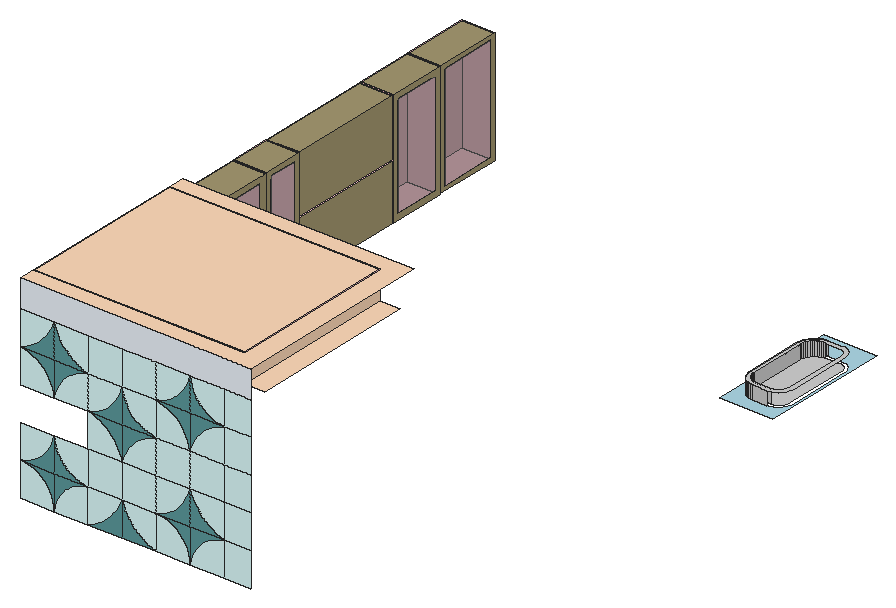
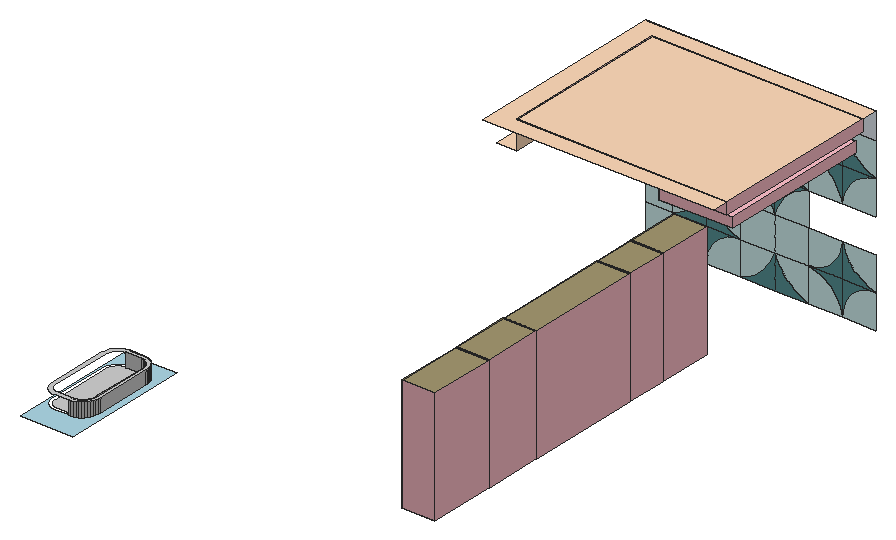
# SketchUp Ruby script. Lengths in inches.
U = 1.inch
M = Sketchup.active_model
def pt(a) = Geom::Point3d.new(a.map { |v| v * U })
def face(e, loops, mat)
  f = e.add_face(loops[0].map { |a| pt(a) })
  loops[1..].each { |l| e.add_face(l.map { |a| pt(a) }).erase! }
  f.material = f.back_material = mat if mat
  f
end
# faces: each face lists its corners as indices into pts; further lists are holes
def faces(e, pts, list, mat = nil) = list.each { |f| face(e, (f[0].is_a?(Array) ? f : [f]).map { |l| l.map { |i| pts[i] } }, mat) }
# xy, xz, yz: faces in a plane at the given z, y or x. An outline is a flat list of corners, or four numbers for a rectangle; further outlines are holes
def ring(l) = l.size == 4 ? [[l[0], l[1]], [l[2], l[1]], [l[2], l[3]], [l[0], l[3]]] : l.each_slice(2).to_a
def flat(e, list, mat, &to3) = list.each { |f| face(e, (f[0].is_a?(Array) ? f : [f]).map { |l| ring(l).map { |u, v| to3.(u, v) } }, mat) }
def xy(e, z, list, mat = nil) = flat(e, list, mat) { |x, y| [x, y, z] }
def xz(e, y, list, mat = nil) = flat(e, list, mat) { |x, z| [x, y, z] }
def yz(e, x, list, mat = nil) = flat(e, list, mat) { |y, z| [x, y, z] }
def lines(e, pts, list) = list.each { |a, b| e.add_line(pt(pts[a]), pt(pts[b])) }
# prism: a flat outline (further loops are holes) pulled along v
def prism(e, loops, v, mat = nil)
  f = face(e, loops, mat); d = Geom::Vector3d.new(v.map { |x| x * U })
  f.pushpull(f.normal.samedirection?(d) ? d.length : -d.length)
end
def box(e, o, s, mat = nil) = prism(e, [[o, [o[0] + s[0], o[1], o[2]], [o[0] + s[0], o[1] + s[1], o[2]], [o[0], o[1] + s[1], o[2]]]], [0, 0, s[2]], mat)
def at(x, y, z, deg = 0) = Geom::Transformation.translation(pt([x, y, z])) * Geom::Transformation.rotation(ORIGIN, Z_AXIS, deg.degrees)
def axes(o, x, y, z) = Geom::Transformation.new([*x, 0, *y, 0, *z, 0, *pt(o).to_a, 1])
def part(name) = M.definitions.add(name)
# library, detail: a bought-in or finely detailed component or shape, given as its bounding box
def library(name, o, s) = part(name).tap { |d| box(d.entities, o, s) }
def detail(e, o, s) = box(e.add_group.entities, o, s)
def put(e, d, t, mat = nil) = e.add_instance(d, t).tap { |i| i.material = mat if mat }
def group(e, t, mat = nil) = e.add_group.tap { |g| g.transformation = t; g.material = mat if mat }.entities
root = M.entities
M.materials.add("[0006_Pink]").color = [255, 192, 203]
M.materials.add("[0027_PeachPuff]").color = [255, 218, 185]
M.materials.add("[0081_CadetBlue]").color = [95, 158, 160]
M.materials.add("[0090_LightCyan]").color = [224, 255, 255]
M.materials.add("[0093_AliceBlue]").color = [240, 248, 255]
M.materials.add("[0095_LightBlue]").color = [173, 216, 230]
M.materials.add("[Carrera Marble]").color = [207, 207, 207]
M.materials.add("[Translucent Glass Gray]").color = [128, 128, 128]
M.materials["[Translucent Glass Gray]"].alpha = 0.5
M.materials.add("[Wood Lumber ButtJoined]").color = [164, 152, 112]
box(root,[118.5625,343,111.75],[25.9375,54.56,3.75],"[0006_Pink]")
xy(root,60.5,[[[244.5625,486.17,263.2,531.9375],[252.11,491,251.42,491.05,250.75,491.2,250.09,491.4375,249.47,491.77,248.9,492.19,248.38,492.68,247.92,493.24,247.54,493.87,247.24,494.54,247.01,495.25,246.88,495.99,246.83,496.73,246.83,516.85,246.88,517.71,247.04,518.55,247.29,519.36,247.64,520.13,248.08,520.85,248.6,521.49,249.2,522.06,249.86,522.53,250.5625,522.91,251.3125,523.19,252.09,523.36,252.88,523.41,258.18,523.41,258.75,523.37,259.3125,523.25,259.86,523.05,260.37,522.78,260.85,522.43,261.28,522.02,261.66,521.55,261.98,521.03,262.23,520.47,262.41,519.88,262.53,519.27,262.5625,518.65,262.5625,496.67,262.52,495.93,262.39,495.21,262.17,494.5,261.86,493.84,261.48,493.22,261.03,492.66,260.52,492.17,259.95,491.76,259.34,491.43,258.69,491.19,258.02,491.05,257.34,491]]],"[0095_LightBlue]")
xy(root,60.5,[[252.11,492.42,257.34,492.42,257.85,492.45,258.35,492.5625,258.84,492.74,259.3,492.99,259.73,493.3,260.11,493.66,260.45,494.08,260.73,494.54,260.96,495.04,261.125,495.57,261.23,496.12,261.26,496.67,261.26,518.65,261.23,519.09,261.15,519.52,261.03,519.93,260.85,520.32,260.62,520.6875,260.36,521.02,260.05,521.31,259.72,521.55,259.36,521.74,258.97,521.88,258.58,521.97,258.18,522,252.88,522,252.26,521.95,251.65,521.82,251.0625,521.61,250.51,521.31,249.99,520.93,249.53,520.49,249.12,519.98,248.77,519.42,248.5,518.82,248.3,518.18,248.18,517.52,248.14,516.85,248.14,496.73,248.17,496.17,248.27,495.62,248.44,495.08,248.67,494.57,248.96,494.11,249.3,493.68,249.69,493.31,250.125,492.99,250.59,492.74,251.08,492.5625,251.59,492.45]],"[Carrera Marble]")
xy(root,65.34,[[[252.11,491,257.34,491,258.02,491.05,258.69,491.19,259.34,491.43,259.95,491.76,260.52,492.17,261.03,492.66,261.48,493.22,261.86,493.84,262.17,494.5,262.39,495.21,262.52,495.93,262.5625,496.67,262.5625,518.65,262.53,519.27,262.41,519.88,262.23,520.47,261.98,521.03,261.66,521.55,261.28,522.02,260.85,522.43,260.37,522.78,259.86,523.05,259.3125,523.25,258.75,523.37,258.18,523.41,252.88,523.41,252.09,523.36,251.3125,523.19,250.5625,522.91,249.86,522.53,249.2,522.06,248.6,521.49,248.08,520.85,247.64,520.13,247.29,519.36,247.04,518.55,246.88,517.71,246.83,516.85,246.83,496.73,246.88,495.99,247.01,495.25,247.24,494.54,247.54,493.87,247.92,493.24,248.38,492.68,248.9,492.19,249.47,491.77,250.09,491.4375,250.75,491.2,251.42,491.05],[252.11,492.42,251.59,492.45,251.08,492.5625,250.59,492.74,250.125,492.99,249.69,493.31,249.3,493.68,248.96,494.11,248.67,494.57,248.44,495.08,248.27,495.62,248.17,496.17,248.14,496.73,248.14,516.85,248.18,517.52,248.3,518.18,248.5,518.82,248.77,519.42,249.12,519.98,249.53,520.49,249.99,520.93,250.51,521.31,251.0625,521.61,251.65,521.82,252.26,521.95,252.88,522,258.18,522,258.58,521.97,258.97,521.88,259.36,521.74,259.72,521.55,260.05,521.31,260.36,521.02,260.62,520.6875,260.85,520.32,261.03,519.93,261.15,519.52,261.23,519.09,261.26,518.65,261.26,496.67,261.23,496.12,261.125,495.57,260.96,495.04,260.73,494.54,260.45,494.08,260.11,493.66,259.73,493.3,259.3,492.99,258.84,492.74,258.35,492.5625,257.85,492.45,257.34,492.42]]],"[Carrera Marble]")
xy(root,76.6875,[[130.1875,408.86,118.5625,408.875,118.58,427.81,130.21,427.8],[130.21,428.36,118.5625,428.375,118.58,442.66,130.23,442.64],[130.22,443.12,118.56,443.125,118.58,483.93,130.24,483.92],[130.25,484.43,118.5625,484.4375,118.58,505.08,130.27,505.06]],"[0006_Pink]")
xy(root,76.84,[[118.5625,505.5625,130.26,529.25]],"[0006_Pink]")
xy(root,96.47,[[129.35,443.12,130.22,443.12,130.24,483.92,129.37,483.93]],"[0006_Pink]")
xy(root,96.97,[[129.35,443.12,129.37,483.93,130.24,483.92,130.22,443.12]],"[0006_Pink]")
xy(root,111.25,[[193.07,339.9375,200.19,399.9375]],"[0027_PeachPuff]")
xy(root,116.9375,[[118.5625,339.9375,193.07,399.9375]],"[0006_Pink]")
xy(root,117.25,[[130.1875,408.86,130.21,427.8,118.58,427.81,118.5625,408.875],[130.21,428.36,130.23,442.64,118.58,442.66,118.5625,428.375],[130.22,443.12,130.24,483.92,118.58,483.93,118.56,443.125],[130.25,484.43,130.27,505.06,118.58,505.08,118.5625,484.4375],[118.5625,505.5625,130.26,529.25]],"[Wood Lumber ButtJoined]")
xy(root,121.1875,[[118.5625,333.9375,200.19,333.9375,200.19,405.9375,118.5625,405.9375,118.5625,399.9375,193.07,399.9375,193.07,339.9375,118.5625,339.9375],[118.5625,339.9375,193.07,399.9375]],"[0027_PeachPuff]")
xz(root,333.9375,[[130.5625,51.41,130.5625,63.41,118.5625,63.41,120.14,63.34,121.69,63.05,123.2,62.57,124.62,61.88,125.9375,61.01,127.125,59.97,128.16,58.78,129.03,57.46,129.72,56.04,130.21,54.54,130.49,52.99],[130.5625,51.41,130.83,52.91,131.26,54.37,131.84,55.78,132.59,57.11,133.47,58.35,134.49,59.49,135.62,60.5,136.86,61.39,138.19,62.125,139.6,62.71,141.0625,63.14,142.5625,63.41,130.5625,63.41],[142.5625,51.41,154.5625,51.41,154.5625,63.41,154.01,62.06,153.36,60.75,152.62,59.49,151.79,58.3,150.875,57.16,149.88,56.09,148.8125,55.1,147.68,54.18,146.48,53.35,145.22,52.61,143.91,51.96],[154.5625,51.41,166.5625,51.41,165.18,51.91,163.85,52.52,162.5625,53.23,161.34,54.05,160.18,54.95,159.1,55.95,158.11,57.03,157.2,58.18,156.39,59.41,155.67,60.69,155.0625,62.03,154.5625,63.41],[178.5625,51.41,178.5625,63.41,166.5625,63.41,168.15,63.35,169.71,63.09,171.22,62.61,172.65,61.93,173.98,61.06,175.17,60.02,176.21,58.82,177.08,57.5,177.76,56.0625,178.24,54.55,178.51,52.99],
  [178.5625,51.41,178.9,52.88,179.38,54.3,180,55.68,180.76,56.97,181.65,58.19,182.66,59.31,183.78,60.32,185,61.21,186.3,61.97,187.67,62.59,189.09,63.07,190.5625,63.41,178.5625,63.41],[118.5625,63.41,130.5625,63.41,130.5625,75.41,130.2,73.96,129.6875,72.55,129.05,71.19,128.27,69.91,127.38,68.71,126.375,67.6,125.26,66.59,124.0625,65.7,122.78,64.93,121.42,64.28,120.01,63.78],[130.5625,63.41,142.5625,63.41,141.02,63.57,139.51,63.92,138.05,64.45,136.67,65.16,135.38,66.04,134.22,67.07,133.19,68.23,132.32,69.51,131.61,70.89,131.07,72.35,130.72,73.86,130.5625,75.41],[166.5625,63.41,178.5625,63.41,178.5625,75.41,178.16,73.97,177.63,72.58,176.97,71.25,176.1875,69.98,175.29,68.79,174.29,67.68,173.18,66.68,171.99,65.78,170.73,65,169.39,64.34,168,63.81],[178.5625,63.41,190.5625,63.41,189.19,63.93,187.86,64.55,186.59,65.27,185.37,66.09,184.22,67,183.15,67.99,182.15,69.07,181.24,70.22,180.42,71.43,179.7,72.71,179.08,74.04,178.5625,75.41],
  [154.5625,75.41,154.5625,87.41,142.5625,87.41,143.98,86.97,145.35,86.41,146.67,85.74,147.93,84.94,149.1,84.04,150.2,83.04,151.2,81.95,152.1,80.77,152.89,79.52,153.57,78.2,154.13,76.83],[154.5625,75.41,155.01,76.82,155.59,78.18,156.27,79.49,157.07,80.74,157.97,81.91,158.97,83,160.0625,84,161.23,84.9,162.48,85.7,163.79,86.39,165.15,86.96,166.5625,87.41,154.5625,87.41],[130.5625,87.41,130.5625,99.41,118.5625,99.41,120.09,99.2,121.57,98.81,123.01,98.24,124.36,97.52,125.62,96.64,126.77,95.62,127.79,94.47,128.67,93.21,129.4,91.85,129.96,90.42,130.35,88.93],[130.5625,87.41,130.93,88.86,131.4375,90.27,132.08,91.625,132.85,92.91,133.74,94.11,134.75,95.22,135.86,96.23,137.0625,97.12,138.35,97.89,139.7,98.53,141.11,99.04,142.5625,99.41,130.5625,99.41],[142.5625,87.41,154.5625,87.41,154.5625,99.41,154.18,97.96,153.66,96.5625,153.01,95.22,152.23,93.94,151.34,92.75,150.33,91.64,149.22,90.64,148.03,89.74,146.75,88.96,145.41,88.3125,144.01,87.79],
  [154.5625,87.41,166.5625,87.41,165.0625,87.67,163.6,88.1,162.19,88.69,160.86,89.43,159.62,90.31,158.49,91.33,157.47,92.47,156.59,93.71,155.84,95.04,155.26,96.45,154.83,97.91,154.5625,99.41],[178.5625,87.41,178.5625,99.41,166.5625,99.41,168.0625,99.14,169.53,98.71,170.93,98.125,172.26,97.39,173.5,96.5,174.64,95.49,175.66,94.35,176.54,93.11,177.28,91.78,177.87,90.37,178.3,88.91],[178.5625,87.41,179.03,88.81,179.61,90.16,180.31,91.46,181.11,92.7,182.02,93.87,183.02,94.95,184.1,95.95,185.27,96.86,186.51,97.66,187.81,98.36,189.16,98.94,190.5625,99.41,178.5625,99.41],[118.5625,99.41,130.5625,99.41,130.5625,111.41,130.04,110.04,129.42,108.71,128.7,107.43,127.88,106.22,126.97,105.07,125.98,103.99,124.9,103,123.75,102.09,122.54,101.27,121.26,100.55,119.93,99.93],[130.5625,99.41,142.5625,99.41,141.14,99.84,139.77,100.4,138.45,101.08,137.2,101.87,136.02,102.77,134.93,103.77,133.93,104.87,133.03,106.05,132.23,107.3,131.56,108.62,131,109.99,130.5625,111.41],
  [166.5625,99.41,178.5625,99.41,178.5625,111.41,178.2,109.96,177.6875,108.55,177.05,107.19,176.27,105.91,175.38,104.71,174.375,103.6,173.26,102.59,172.0625,101.7,170.78,100.93,169.42,100.28,168.01,99.78],[178.5625,99.41,190.5625,99.41,189.03,99.6,187.54,99.98,186.1,100.53,184.73,101.25,183.46,102.13,182.31,103.15,181.28,104.31,180.41,105.58,179.6875,106.94,179.13,108.38,178.76,109.88,178.5625,111.41]],"[0081_CadetBlue]")
xz(root,333.9375,[[118.5625,51.41,130.5625,51.41,130.49,52.99,130.21,54.54,129.72,56.04,129.03,57.46,128.16,58.78,127.125,59.97,125.9375,61.01,124.62,61.88,123.2,62.57,121.69,63.05,120.14,63.34,118.5625,63.41],[130.5625,51.41,142.5625,51.41,142.5625,63.41,141.0625,63.14,139.6,62.71,138.19,62.125,136.86,61.39,135.62,60.5,134.49,59.49,133.47,58.35,132.59,57.11,131.84,55.78,131.26,54.37,130.83,52.91],[142.5625,51.41,143.91,51.96,145.22,52.61,146.48,53.35,147.68,54.18,148.8125,55.1,149.88,56.09,150.875,57.16,151.79,58.3,152.62,59.49,153.36,60.75,154.01,62.06,154.5625,63.41,142.5625,63.41],[166.5625,51.41,166.5625,63.41,154.5625,63.41,155.0625,62.03,155.67,60.69,156.39,59.41,157.2,58.18,158.11,57.03,159.1,55.95,160.18,54.95,161.34,54.05,162.5625,53.23,163.85,52.52,165.18,51.91],[166.5625,51.41,178.5625,51.41,178.51,52.99,178.24,54.55,177.76,56.0625,177.08,57.5,176.21,58.82,175.17,60.02,173.98,61.06,172.65,61.93,171.22,62.61,169.71,63.09,168.15,63.35,166.5625,63.41],
  [178.5625,51.41,190.5625,51.41,190.5625,63.41,189.09,63.07,187.67,62.59,186.3,61.97,185,61.21,183.78,60.32,182.66,59.31,181.65,58.19,180.76,56.97,180,55.68,179.38,54.3,178.9,52.88],[190.5625,51.41,200.19,63.41],[118.5625,63.41,120.01,63.78,121.42,64.28,122.78,64.93,124.0625,65.7,125.26,66.59,126.375,67.6,127.38,68.71,128.27,69.91,129.05,71.19,129.6875,72.55,130.2,73.96,130.5625,75.41,118.5625,75.41],[142.5625,63.41,142.5625,75.41,130.5625,75.41,130.72,73.86,131.07,72.35,131.61,70.89,132.32,69.51,133.19,68.23,134.22,67.07,135.38,66.04,136.67,65.16,138.05,64.45,139.51,63.92,141.02,63.57],[142.5625,63.41,154.5625,75.41],
  [154.5625,63.41,166.5625,75.41],[166.5625,63.41,168,63.81,169.39,64.34,170.73,65,171.99,65.78,173.18,66.68,174.29,67.68,175.29,68.79,176.1875,69.98,176.97,71.25,177.63,72.58,178.16,73.97,178.5625,75.41,166.5625,75.41],[190.5625,63.41,190.5625,75.41,178.5625,75.41,179.08,74.04,179.7,72.71,180.42,71.43,181.24,70.22,182.15,69.07,183.15,67.99,184.22,67,185.37,66.09,186.59,65.27,187.86,64.55,189.19,63.93],[190.5625,63.41,200.19,75.41],[142.5625,75.41,154.5625,75.41,154.13,76.83,153.57,78.2,152.89,79.52,152.1,80.77,151.2,81.95,150.2,83.04,149.1,84.04,147.93,84.94,146.67,85.74,145.35,86.41,143.98,86.97,142.5625,87.41],
  [154.5625,75.41,166.5625,75.41,166.5625,87.41,165.15,86.96,163.79,86.39,162.48,85.7,161.23,84.9,160.0625,84,158.97,83,157.97,81.91,157.07,80.74,156.27,79.49,155.59,78.18,155.01,76.82],[166.5625,75.41,178.5625,87.41],[178.5625,75.41,190.5625,87.41],[190.5625,75.41,200.19,87.41],[118.5625,87.41,130.5625,87.41,130.35,88.93,129.96,90.42,129.4,91.85,128.67,93.21,127.79,94.47,126.77,95.62,125.62,96.64,124.36,97.52,123.01,98.24,121.57,98.81,120.09,99.2,118.5625,99.41],
  [130.5625,87.41,142.5625,87.41,142.5625,99.41,141.11,99.04,139.7,98.53,138.35,97.89,137.0625,97.12,135.86,96.23,134.75,95.22,133.74,94.11,132.85,92.91,132.08,91.625,131.4375,90.27,130.93,88.86],[142.5625,87.41,144.01,87.79,145.41,88.3125,146.75,88.96,148.03,89.74,149.22,90.64,150.33,91.64,151.34,92.75,152.23,93.94,153.01,95.22,153.66,96.5625,154.18,97.96,154.5625,99.41,142.5625,99.41],[166.5625,87.41,166.5625,99.41,154.5625,99.41,154.83,97.91,155.26,96.45,155.84,95.04,156.59,93.71,157.47,92.47,158.49,91.33,159.62,90.31,160.86,89.43,162.19,88.69,163.6,88.1,165.0625,87.67],[166.5625,87.41,178.5625,87.41,178.3,88.91,177.87,90.37,177.28,91.78,176.54,93.11,175.66,94.35,174.64,95.49,173.5,96.5,172.26,97.39,170.93,98.125,169.53,98.71,168.0625,99.14,166.5625,99.41],[178.5625,87.41,190.5625,87.41,190.5625,99.41,189.16,98.94,187.81,98.36,186.51,97.66,185.27,96.86,184.1,95.95,183.02,94.95,182.02,93.87,181.11,92.7,180.31,91.46,179.61,90.16,179.03,88.81],
  [190.5625,87.41,200.19,99.41],[118.5625,99.41,119.93,99.93,121.26,100.55,122.54,101.27,123.75,102.09,124.9,103,125.98,103.99,126.97,105.07,127.88,106.22,128.7,107.43,129.42,108.71,130.04,110.04,130.5625,111.41,118.5625,111.41],[142.5625,99.41,142.5625,111.41,130.5625,111.41,131,109.99,131.56,108.62,132.23,107.3,133.03,106.05,133.93,104.87,134.93,103.77,136.02,102.77,137.2,101.87,138.45,101.08,139.77,100.4,141.14,99.84],[142.5625,99.41,154.5625,111.41],[154.5625,99.41,166.5625,111.41],
  [166.5625,99.41,168.01,99.78,169.42,100.28,170.78,100.93,172.0625,101.7,173.26,102.59,174.375,103.6,175.38,104.71,176.27,105.91,177.05,107.19,177.6875,108.55,178.2,109.96,178.5625,111.41,166.5625,111.41],[190.5625,99.41,190.5625,111.41,178.5625,111.41,178.76,109.88,179.13,108.38,179.6875,106.94,180.41,105.58,181.28,104.31,182.31,103.15,183.46,102.13,184.73,101.25,186.1,100.53,187.54,99.98,189.03,99.6],[190.5625,99.41,200.19,111.41]],"[0090_LightCyan]")
xz(root,333.9375,[[118.5625,111.41,200.19,121.1875]],"[0093_AliceBlue]")
xz(root,339.9375,[[118.5625,116.9375,193.07,121.1875]],"[0006_Pink]")
xz(root,399.9375,[[118.5625,116.9375,193.07,121.1875]],"[0006_Pink]")
xz(root,491,[[252.11,60.5,257.34,65.34]],"[Carrera Marble]")
xz(root,492.42,[[252.11,60.5,257.34,65.34]],"[Carrera Marble]")
xz(root,505.5625,[[118.5625,76.84,130.26,117.25]],"[0006_Pink]")
xz(root,529.25,[[118.5625,76.84,130.26,117.25]],"[0006_Pink]")
yz(root,118.5625,[[505.5625,76.84,529.25,117.25],[339.9375,116.9375,399.9375,121.1875]],"[0006_Pink]")
yz(root,130.26,[[507.08,78.36,527.73,115.73]],"[Translucent Glass Gray]")
yz(root,130.26,[[[505.5625,76.84,529.25,117.25],[507.08,78.36,527.73,115.73]]],"[Wood Lumber ButtJoined]")
yz(root,193.07,[[339.9375,116.9375,399.9375,121.1875]],"[0006_Pink]")
yz(root,193.07,[[339.9375,111.25,399.9375,121.1875]],"[0027_PeachPuff]")
yz(root,246.83,[[496.73,60.5,516.85,65.34]],"[Carrera Marble]")
yz(root,248.14,[[496.73,60.5,516.85,65.34]],"[Carrera Marble]")
p = [[250.75,491.2,60.5],[251.42,491.05,60.5],[251.42,491.05,65.34],[250.75,491.2,65.34],[252.11,491,60.5],[252.11,491,65.34],
  [250.09,491.4375,60.5],[250.09,491.4375,65.34],[249.47,491.77,60.5],[249.47,491.77,65.34],[248.9,492.19,60.5],[248.9,492.19,65.34],
  [248.38,492.68,60.5],[248.38,492.68,65.34],[252.11,492.42,60.5],[251.59,492.45,60.5],[251.59,492.45,65.34],[252.11,492.42,65.34],
  [251.08,492.5625,60.5],[251.08,492.5625,65.34],[250.59,492.74,60.5],[250.59,492.74,65.34],[247.92,493.24,60.5],[247.92,493.24,65.34],
  [250.125,492.99,60.5],[250.125,492.99,65.34],[249.69,493.31,60.5],[249.69,493.31,65.34],[247.54,493.87,60.5],[247.54,493.87,65.34],
  [249.3,493.68,60.5],[249.3,493.68,65.34],[248.96,494.11,60.5],[248.96,494.11,65.34],[247.24,494.54,60.5],[247.24,494.54,65.34],
  [248.67,494.57,60.5],[248.67,494.57,65.34],[247.01,495.25,60.5],[247.01,495.25,65.34],[248.44,495.08,60.5],[248.44,495.08,65.34],
  [248.27,495.62,60.5],[248.27,495.62,65.34],[246.88,495.99,60.5],[246.88,495.99,65.34],[248.17,496.17,60.5],[248.17,496.17,65.34],
  [246.83,496.73,60.5],[246.83,496.73,65.34],[248.14,496.73,60.5],[248.14,496.73,65.34],[246.88,517.71,60.5],[246.83,516.85,60.5],
  [246.83,516.85,65.34],[246.88,517.71,65.34],[248.14,516.85,60.5],[248.18,517.52,60.5],[248.18,517.52,65.34],[248.14,516.85,65.34],
  [248.3,518.18,60.5],[248.3,518.18,65.34],[247.04,518.55,60.5],[247.04,518.55,65.34],[248.5,518.82,60.5],[248.5,518.82,65.34],
  [247.29,519.36,60.5],[247.29,519.36,65.34],[248.77,519.42,60.5],[248.77,519.42,65.34],[247.64,520.13,60.5],[247.64,520.13,65.34],
  [249.12,519.98,60.5],[249.12,519.98,65.34],[249.53,520.49,60.5],[249.53,520.49,65.34],[248.08,520.85,60.5],[248.08,520.85,65.34],
  [249.99,520.93,60.5],[249.99,520.93,65.34],[248.6,521.49,60.5],[248.6,521.49,65.34],[250.51,521.31,60.5],[250.51,521.31,65.34],
  [251.0625,521.61,60.5],[251.0625,521.61,65.34],[249.2,522.06,60.5],[249.2,522.06,65.34],[251.65,521.82,60.5],[251.65,521.82,65.34],
  [252.26,521.95,60.5],[252.26,521.95,65.34],[252.88,522,60.5],[252.88,522,65.34],[249.86,522.53,60.5],[249.86,522.53,65.34],
  [250.5625,522.91,60.5],[250.5625,522.91,65.34],[251.3125,523.19,60.5],[251.3125,523.19,65.34],[252.09,523.36,60.5],[252.09,523.36,65.34],
  [252.88,523.41,60.5],[252.88,523.41,65.34],[118.5625,408.875,117.25],[118.58,427.81,117.25],[118.58,427.81,76.6875],[118.5625,408.875,76.6875],
  [130.1875,408.86,76.6875],[130.1875,408.86,117.25],[130.21,427.8,117.25],[130.21,427.8,76.6875],[130.2,425.56,115.01],[130.2,425.56,78.93],
  [130.19,411.1,78.93],[130.19,411.1,115.01],[118.58,442.66,76.6875],[118.5625,428.375,76.6875],[118.5625,428.375,117.25],[118.58,442.66,117.25],
  [130.21,428.36,76.6875],[130.21,428.36,117.25],[130.23,442.64,76.6875],[130.23,442.64,117.25],[130.21,430.39,78.72],[130.21,430.39,115.22],
  [130.23,440.61,115.22],[130.23,440.61,78.72],[118.58,483.93,117.25],[118.58,483.93,76.6875],[118.56,443.125,76.6875],[118.56,443.125,117.25],
  [130.22,443.12,76.6875],[130.22,443.12,96.47],[129.35,443.12,96.47],[129.35,443.12,96.97],[130.22,443.12,96.97],[130.22,443.12,117.25],
  [130.24,483.92,76.6875],[130.24,483.92,96.47],[130.24,483.92,117.25],[130.24,483.92,96.97],[129.37,483.93,96.97],[129.37,483.93,96.47],
  [118.5625,484.4375,117.25],[118.58,505.08,117.25],[118.58,505.08,76.6875],[118.5625,484.4375,76.6875],[130.25,484.43,76.6875],[130.25,484.43,117.25],
  [130.27,505.06,117.25],[130.27,505.06,76.6875],[130.25,486.37,78.63],[130.25,486.37,115.3],[130.26,503.12,115.3],[130.26,503.12,78.63]]
faces(root,p,[[0,1,2,3],[1,4,5,2],[6,0,3,7],[8,6,7,9],[10,8,9,11],[12,10,11,13],[14,15,16,17],[15,18,19,16],
  [18,20,21,19],[22,12,13,23],[20,24,25,21],[24,26,27,25],[28,22,23,29],[26,30,31,27],[30,32,33,31],[34,28,29,35],
  [32,36,37,33],[38,34,35,39],[36,40,41,37],[40,42,43,41],[44,38,39,45],[42,46,47,43],[48,44,45,49],[46,50,51,47],
  [52,53,54,55],[56,57,58,59],[57,60,61,58],[62,52,55,63],[60,64,65,61],[66,62,63,67],[64,68,69,65],[70,66,67,71],
  [68,72,73,69],[72,74,75,73],[76,70,71,77],[74,78,79,75],[80,76,77,81],[78,82,83,79],[82,84,85,83],[86,80,81,87],
  [84,88,89,85],[88,90,91,89],[90,92,93,91],[94,86,87,95],[96,94,95,97],[98,96,97,99],[100,98,99,101],[102,100,101,103]],"[Carrera Marble]")
faces(root,p,[[104,105,106,107],[104,107,108,109],[106,105,110,111],[116,117,118,119],[118,117,120,121],[116,119,123,122],[128,129,130,131],[132,133,134,135,136,137,131,130],
  [140,141,142,143,139,138,129,128],[144,145,146,147],[144,147,148,149],[146,145,150,151],[135,134,143,142]],"[0006_Pink]")
faces(root,p,[[[110,109,108,111],[112,113,114,115]],[[120,122,123,121],[124,125,126,127]],[138,139,133,132],[[150,149,148,151],[152,153,154,155]],[137,136,141,140]],"[Wood Lumber ButtJoined]")
faces(root,p,[[153,152,155,154],[125,124,127,126],[113,112,115,114]],"[Translucent Glass Gray]")
